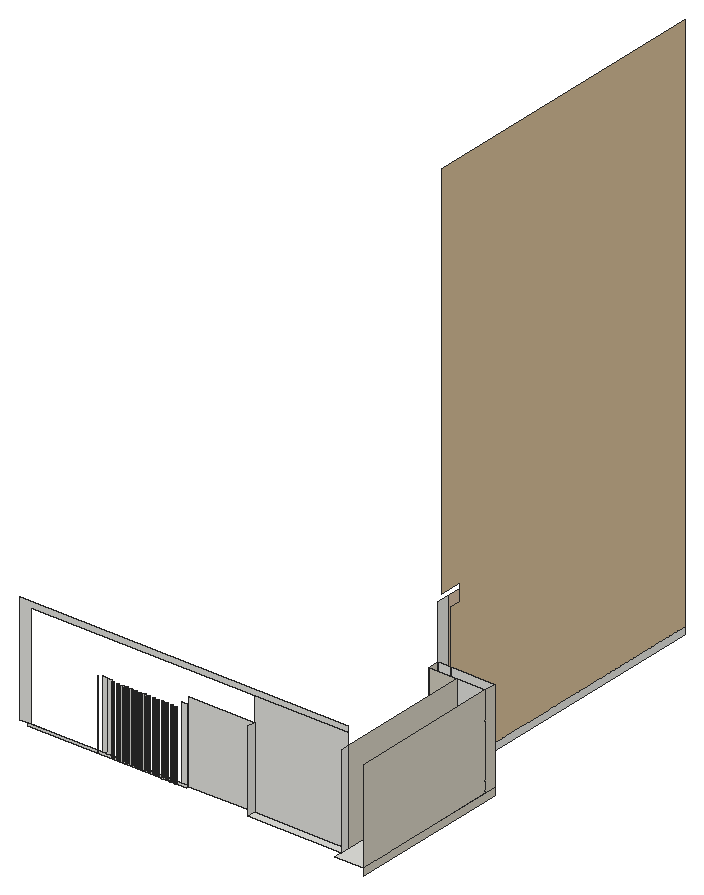
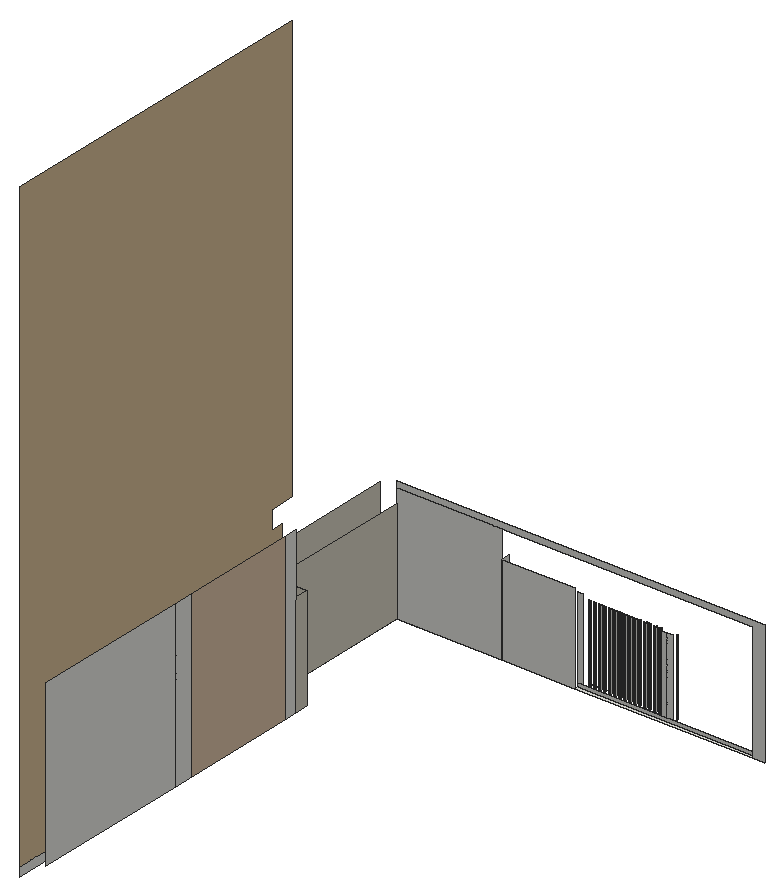
# SketchUp Ruby script. Lengths in inches.
U = 1.inch
M = Sketchup.active_model
def pt(a) = Geom::Point3d.new(a.map { |v| v * U })
def face(e, loops, mat)
  f = e.add_face(loops[0].map { |a| pt(a) })
  loops[1..].each { |l| e.add_face(l.map { |a| pt(a) }).erase! }
  f.material = f.back_material = mat if mat
  f
end
# faces: each face lists its corners as indices into pts; further lists are holes
def faces(e, pts, list, mat = nil) = list.each { |f| face(e, (f[0].is_a?(Array) ? f : [f]).map { |l| l.map { |i| pts[i] } }, mat) }
# xy, xz, yz: faces in a plane at the given z, y or x. An outline is a flat list of corners, or four numbers for a rectangle; further outlines are holes
def ring(l) = l.size == 4 ? [[l[0], l[1]], [l[2], l[1]], [l[2], l[3]], [l[0], l[3]]] : l.each_slice(2).to_a
def flat(e, list, mat, &to3) = list.each { |f| face(e, (f[0].is_a?(Array) ? f : [f]).map { |l| ring(l).map { |u, v| to3.(u, v) } }, mat) }
def xy(e, z, list, mat = nil) = flat(e, list, mat) { |x, y| [x, y, z] }
def xz(e, y, list, mat = nil) = flat(e, list, mat) { |x, z| [x, y, z] }
def yz(e, x, list, mat = nil) = flat(e, list, mat) { |y, z| [x, y, z] }
def lines(e, pts, list) = list.each { |a, b| e.add_line(pt(pts[a]), pt(pts[b])) }
# prism: a flat outline (further loops are holes) pulled along v
def prism(e, loops, v, mat = nil)
  f = face(e, loops, mat); d = Geom::Vector3d.new(v.map { |x| x * U })
  f.pushpull(f.normal.samedirection?(d) ? d.length : -d.length)
end
def box(e, o, s, mat = nil) = prism(e, [[o, [o[0] + s[0], o[1], o[2]], [o[0] + s[0], o[1] + s[1], o[2]], [o[0], o[1] + s[1], o[2]]]], [0, 0, s[2]], mat)
def at(x, y, z, deg = 0) = Geom::Transformation.translation(pt([x, y, z])) * Geom::Transformation.rotation(ORIGIN, Z_AXIS, deg.degrees)
def axes(o, x, y, z) = Geom::Transformation.new([*x, 0, *y, 0, *z, 0, *pt(o).to_a, 1])
def part(name) = M.definitions.add(name)
# library, detail: a bought-in or finely detailed component or shape, given as its bounding box
def library(name, o, s) = part(name).tap { |d| box(d.entities, o, s) }
def detail(e, o, s) = box(e.add_group.entities, o, s)
def put(e, d, t, mat = nil) = e.add_instance(d, t).tap { |i| i.material = mat if mat }
def group(e, t, mat = nil) = e.add_group.tap { |g| g.transformation = t; g.material = mat if mat }.entities
root = M.entities
M.materials.add("[Formica Beige]").color = [211, 187, 149]
M.materials.add("[Formica Graystone]").color = [209, 204, 189]
M.materials.add("[Formica Laminate Light]").color = [213, 189, 164]
xy(root,9,[[762.14,1.67,797.12,189.01],[646.62,11.52,762.14,21.38],[370.65,17.41,566.39,21.38],[727.17,189.01,797.12,203.79]])
xy(root,12.5,[[539.51,12.51,539.19,12.55,538.89,12.67,538.63,12.875,538.43,13.13,538.31,13.43,538.26,13.76,538.31,14.08,538.43,14.38,538.63,14.64,538.89,14.84,539.19,14.96,539.51,15.01,539.84,14.96,540.14,14.84,540.4,14.64,540.6,14.38,540.72,14.08,540.76,13.76,540.72,13.43,540.6,13.13,540.4,12.875,540.14,12.67,539.84,12.55],[544.76,12.51,544.44,12.55,544.14,12.67,543.88,12.875,543.68,13.13,543.56,13.43,543.51,13.76,543.56,14.08,543.68,14.38,543.88,14.64,544.14,14.84,544.44,14.96,544.76,15.01,545.09,14.96,545.39,14.84,545.65,14.64,545.85,14.38,545.97,14.08,546.01,13.76,545.97,13.43,545.85,13.13,545.65,12.875,545.39,12.67,545.09,12.55],[550.39,12.51,550.07,12.55,549.76,12.67,549.51,12.875,549.31,13.13,549.18,13.43,549.14,13.76,549.18,14.08,549.31,14.38,549.51,14.64,549.76,14.84,550.07,14.96,550.39,15.01,550.71,14.96,551.01,14.84,551.27,14.64,551.47,14.38,551.6,14.08,551.64,13.76,551.6,13.43,551.47,13.13,551.27,12.875,551.01,12.67,550.71,12.55],[555.89,12.51,555.57,12.55,555.26,12.67,555.01,12.875,554.81,13.13,554.68,13.43,554.64,13.76,554.68,14.08,554.81,14.38,555.01,14.64,555.26,14.84,555.57,14.96,555.89,15.01,556.21,14.96,556.51,14.84,556.77,14.64,556.97,14.38,557.1,14.08,557.14,13.76,557.1,13.43,556.97,13.13,556.77,12.875,556.51,12.67,556.21,12.55]])
xz(root,17.41,[[370.65,9,566.39,12.5],[462.5,12.5,468.46,96.37],[468.46,12.5,474.42,96.37],[560.77,12.5,566.39,102.25]])
xz(root,21.38,[[357.9375,9,357.9375,145.125,762.14,145.125,762.14,138.11,370.65,138.11,370.65,9],[566.39,9,646.62,108],[646.62,9,762.14,138.11]])
xz(root,189.01,[[762.14,9,797.12,122.6875]])
xz(root,189.01,[[727.17,9,762.14,122.6875]],"[Formica Graystone]")
xz(root,203.79,[[742.93,0,797.12,9],[727.17,9,742.93,122.6875],[742.93,9,797.12,122.6875]])
yz(root,646.62,[[11.52,9,21.38,108]])
yz(root,727.17,[[203.79,9,219.56,189],[348.07,9,370.07,189],[370.07,9,548.03,189]])
yz(root,727.17,[[189.01,9,203.79,122.6875]],"[Formica Graystone]")
yz(root,727.17,[[219.56,9,348.07,189]],"[Formica Laminate Light]")
yz(root,742.93,[[203.79,0,563.79,9]])
yz(root,742.93,[[203.79,9,563.79,9,563.79,679.64,190.11,679.64,190.11,209.5,218.11,209.5,218.11,189,203.79,189]],"[Formica Beige]")
yz(root,762.14,[[11.52,9,21.38,122.6875]])
yz(root,762.14,[[21.38,9,189.01,122.6875]],"[Formica Graystone]")
yz(root,797.12,[[1.67,0,203.79,9],[1.67,9,189.01,122.6875],[189.01,9,203.79,122.6875]],"[Formica Graystone]")
p = [[459.89,13.76,12.5],[459.85,14.08,12.5],[459.85,14.08,96.37],[459.89,13.76,96.37],[477.24,14.08,12.5],[477.2,13.76,12.5],
  [477.2,13.76,96.37],[477.24,14.08,96.37],[479.7,13.76,12.5],[479.66,14.08,12.5],[479.66,14.08,96.37],[479.7,13.76,96.37],
  [482.81,14.08,12.5],[482.76,13.76,12.5],[482.76,13.76,96.37],[482.81,14.08,96.37],[485.26,13.76,12.5],[485.22,14.08,12.5],
  [485.22,14.08,96.37],[485.26,13.76,96.37],[488.62,14.08,12.5],[488.58,13.76,12.5],[488.58,13.76,96.37],[488.62,14.08,96.37],
  [491.08,13.76,12.5],[491.03,14.08,12.5],[491.03,14.08,96.37],[491.08,13.76,96.37],[493.93,14.08,12.5],[493.89,13.76,12.5],
  [493.89,13.76,96.37],[493.93,14.08,96.37],[496.39,13.76,12.5],[496.35,14.08,12.5],[496.35,14.08,96.37],[496.39,13.76,96.37],
  [499.74,14.08,12.5],[499.7,13.76,12.5],[499.7,13.76,96.37],[499.74,14.08,96.37],[502.2,13.76,12.5],[502.16,14.08,12.5],
  [502.16,14.08,96.37],[502.2,13.76,96.37],[504.87,14.08,12.5],[504.83,13.76,12.5],[504.83,13.76,96.37],[504.87,14.08,96.37],
  [507.33,13.76,12.5],[507.28,14.08,12.5],[507.28,14.08,96.37],[507.33,13.76,96.37],[510.49,14.08,12.5],[510.45,13.76,12.5],
  [510.45,13.76,96.37],[510.49,14.08,96.37],[512.95,13.76,12.5],[512.91,14.08,12.5],[512.91,14.08,96.37],[512.95,13.76,96.37],
  [515.81,14.08,12.5],[515.76,13.76,12.5],[515.76,13.76,96.37],[515.81,14.08,96.37],[518.26,13.76,12.5],[518.22,14.08,12.5],
  [518.22,14.08,96.37],[518.26,13.76,96.37],[521.12,14.08,12.5],[521.08,13.76,12.5],[521.08,13.76,96.37],[521.12,14.08,96.37],
  [523.58,13.76,12.5],[523.53,14.08,12.5],[523.53,14.08,96.37],[523.58,13.76,96.37],[526.99,14.08,12.5],[526.95,13.76,12.5],
  [526.95,13.76,96.37],[526.99,14.08,96.37],[529.45,13.76,12.5],[529.41,14.08,12.5],[529.41,14.08,96.37],[529.45,13.76,96.37],
  [532.49,14.08,12.5],[532.45,13.76,12.5],[532.45,13.76,96.37],[532.49,14.08,96.37],[534.95,13.76,12.5],[534.91,14.08,12.5],
  [534.91,14.08,96.37],[534.95,13.76,96.37],[538.31,14.08,12.5],[538.26,13.76,12.5],[538.26,13.76,96.37],[538.31,14.08,96.37],
  [540.76,13.76,12.5],[540.72,14.08,12.5],[540.72,14.08,96.37],[540.76,13.76,96.37],[543.56,14.08,12.5],[543.51,13.76,12.5],
  [543.51,13.76,96.37],[543.56,14.08,96.37],[546.01,13.76,12.5],[545.97,14.08,12.5],[545.97,14.08,96.37],[546.01,13.76,96.37],
  [549.18,14.08,12.5],[549.14,13.76,12.5],[549.14,13.76,96.37],[549.18,14.08,96.37],[551.64,13.76,12.5],[551.6,14.08,12.5],
  [551.6,14.08,96.37],[551.64,13.76,96.37],[554.68,14.08,12.5],[554.64,13.76,12.5],[554.64,13.76,96.37],[554.68,14.08,96.37],
  [557.14,13.76,12.5],[557.1,14.08,12.5],[557.1,14.08,96.37],[557.14,13.76,96.37],[459.72,14.38,12.5],[459.72,14.38,96.37],
  [477.37,14.38,12.5],[477.37,14.38,96.37],[479.53,14.38,12.5],[479.53,14.38,96.37],[482.93,14.38,12.5],[482.93,14.38,96.37],
  [485.1,14.38,12.5],[485.1,14.38,96.37],[488.74,14.38,12.5],[488.74,14.38,96.37],[490.91,14.38,12.5],[490.91,14.38,96.37],
  [494.06,14.38,12.5],[494.06,14.38,96.37],[496.22,14.38,12.5],[496.22,14.38,96.37],[499.87,14.38,12.5],[499.87,14.38,96.37],
  [502.03,14.38,12.5],[502.03,14.38,96.37],[504.99,14.38,12.5],[504.99,14.38,96.37],[507.16,14.38,12.5],[507.16,14.38,96.37],
  [510.62,14.38,12.5],[510.62,14.38,96.37],[512.78,14.38,12.5],[512.78,14.38,96.37],[515.93,14.38,12.5],[515.93,14.38,96.37],
  [518.1,14.38,12.5],[518.1,14.38,96.37],[521.24,14.38,12.5],[521.24,14.38,96.37],[523.41,14.38,12.5],[523.41,14.38,96.37],
  [527.12,14.38,12.5],[527.12,14.38,96.37],[529.28,14.38,12.5],[529.28,14.38,96.37],[532.62,14.38,12.5],[532.62,14.38,96.37],
  [534.78,14.38,12.5],[534.78,14.38,96.37],[538.43,14.38,12.5],[538.43,14.38,96.37],[540.6,14.38,12.5],[540.6,14.38,96.37],
  [543.68,14.38,12.5],[543.68,14.38,96.37],[545.85,14.38,12.5],[545.85,14.38,96.37],[549.31,14.38,12.5],[549.31,14.38,96.37],
  [551.47,14.38,12.5],[551.47,14.38,96.37],[554.81,14.38,12.5],[554.81,14.38,96.37],[556.97,14.38,12.5],[556.97,14.38,96.37],
  [477.57,14.64,12.5],[477.57,14.64,96.37],[479.34,14.64,12.5],[479.34,14.64,96.37],[483.13,14.64,12.5],[483.13,14.64,96.37],
  [484.9,14.64,12.5],[484.9,14.64,96.37],[488.94,14.64,12.5],[488.94,14.64,96.37],[490.71,14.64,12.5],[490.71,14.64,96.37],
  [494.26,14.64,12.5],[494.26,14.64,96.37],[496.02,14.64,12.5],[496.02,14.64,96.37],[500.07,14.64,12.5],[500.07,14.64,96.37],
  [501.84,14.64,12.5],[501.84,14.64,96.37],[505.19,14.64,12.5],[505.19,14.64,96.37],[506.96,14.64,12.5],[506.96,14.64,96.37],
  [510.82,14.64,12.5],[510.82,14.64,96.37],[512.59,14.64,12.5],[512.59,14.64,96.37],[516.13,14.64,12.5],[516.13,14.64,96.37],
  [517.9,14.64,12.5],[517.9,14.64,96.37],[521.44,14.64,12.5],[521.44,14.64,96.37],[523.21,14.64,12.5],[523.21,14.64,96.37],
  [527.32,14.64,12.5],[527.32,14.64,96.37],[529.09,14.64,12.5],[529.09,14.64,96.37],[532.82,14.64,12.5],[532.82,14.64,96.37],
  [534.59,14.64,12.5],[534.59,14.64,96.37],[538.63,14.64,12.5],[538.63,14.64,96.37],[540.4,14.64,12.5],[540.4,14.64,96.37],
  [543.88,14.64,12.5],[543.88,14.64,96.37],[545.65,14.64,12.5],[545.65,14.64,96.37],[549.51,14.64,12.5],[549.51,14.64,96.37],
  [551.27,14.64,12.5],[551.27,14.64,96.37],[555.01,14.64,12.5],[555.01,14.64,96.37],[556.77,14.64,12.5],[556.77,14.64,96.37],
  [477.83,14.84,12.5],[477.83,14.84,96.37],[479.08,14.84,12.5],[479.08,14.84,96.37],[483.39,14.84,12.5],[483.39,14.84,96.37],
  [484.64,14.84,12.5],[484.64,14.84,96.37],[489.2,14.84,12.5],[489.2,14.84,96.37],[490.45,14.84,12.5],[490.45,14.84,96.37],
  [494.51,14.84,12.5],[494.51,14.84,96.37],[495.76,14.84,12.5],[495.76,14.84,96.37],[500.33,14.84,12.5],[500.33,14.84,96.37],
  [501.58,14.84,12.5],[501.58,14.84,96.37],[505.45,14.84,12.5],[505.45,14.84,96.37],[506.7,14.84,12.5],[506.7,14.84,96.37],
  [511.08,14.84,12.5],[511.08,14.84,96.37],[512.33,14.84,12.5],[512.33,14.84,96.37],[516.39,14.84,12.5],[516.39,14.84,96.37],
  [517.64,14.84,12.5],[517.64,14.84,96.37],[521.7,14.84,12.5],[521.7,14.84,96.37],[522.95,14.84,12.5],[522.95,14.84,96.37],
  [527.58,14.84,12.5],[527.58,14.84,96.37],[528.83,14.84,12.5],[528.83,14.84,96.37],[533.08,14.84,12.5],[533.08,14.84,96.37],
  [534.33,14.84,12.5],[534.33,14.84,96.37],[538.89,14.84,12.5],[538.89,14.84,96.37],[540.14,14.84,12.5],[540.14,14.84,96.37],
  [544.14,14.84,12.5],[544.14,14.84,96.37],[545.39,14.84,12.5],[545.39,14.84,96.37],[549.76,14.84,12.5],[549.76,14.84,96.37],
  [551.01,14.84,12.5],[551.01,14.84,96.37],[555.26,14.84,12.5],[555.26,14.84,96.37],[556.51,14.84,12.5],[556.51,14.84,96.37],
  [478.13,14.96,12.5],[478.13,14.96,96.37],[478.78,14.96,12.5],[478.78,14.96,96.37],[483.69,14.96,12.5],[483.69,14.96,96.37],
  [484.34,14.96,12.5],[484.34,14.96,96.37],[489.5,14.96,12.5],[489.5,14.96,96.37],[490.15,14.96,12.5],[490.15,14.96,96.37],
  [494.82,14.96,12.5],[494.82,14.96,96.37],[495.46,14.96,12.5],[495.46,14.96,96.37],[500.63,14.96,12.5],[500.63,14.96,96.37],
  [501.28,14.96,12.5],[501.28,14.96,96.37],[505.75,14.96,12.5],[505.75,14.96,96.37],[506.4,14.96,12.5],[506.4,14.96,96.37],
  [511.38,14.96,12.5],[511.38,14.96,96.37],[512.03,14.96,12.5],[512.03,14.96,96.37],[516.69,14.96,12.5],[516.69,14.96,96.37],
  [517.34,14.96,12.5],[517.34,14.96,96.37],[522,14.96,12.5],[522,14.96,96.37],[522.65,14.96,12.5],[522.65,14.96,96.37],
  [527.88,14.96,12.5],[527.88,14.96,96.37],[528.53,14.96,12.5],[528.53,14.96,96.37],[533.38,14.96,12.5],[533.38,14.96,96.37],
  [534.03,14.96,12.5],[534.03,14.96,96.37],[539.19,14.96,12.5],[539.19,14.96,96.37],[539.84,14.96,12.5],[539.84,14.96,96.37],
  [544.44,14.96,12.5],[544.44,14.96,96.37],[545.09,14.96,12.5],[545.09,14.96,96.37],[550.07,14.96,12.5],[550.07,14.96,96.37],
  [550.71,14.96,12.5],[550.71,14.96,96.37],[555.57,14.96,12.5],[555.57,14.96,96.37],[556.21,14.96,12.5],[556.21,14.96,96.37],
  [478.45,15.01,12.5],[478.45,15.01,96.37],[484.01,15.01,12.5],[484.01,15.01,96.37],[489.83,15.01,12.5],[489.83,15.01,96.37],
  [495.14,15.01,12.5],[495.14,15.01,96.37],[500.95,15.01,12.5],[500.95,15.01,96.37],[506.08,15.01,12.5],[506.08,15.01,96.37],
  [511.7,15.01,12.5],[511.7,15.01,96.37],[517.01,15.01,12.5],[517.01,15.01,96.37],[522.33,15.01,12.5],[522.33,15.01,96.37],
  [528.2,15.01,12.5],[528.2,15.01,96.37],[533.7,15.01,12.5],[533.7,15.01,96.37],[539.51,15.01,12.5],[539.51,15.01,96.37],
  [544.76,15.01,12.5],[544.76,15.01,96.37],[550.39,15.01,12.5],[550.39,15.01,96.37],[555.89,15.01,12.5],[555.89,15.01,96.37]]
faces(root,p,[[0,1,2,3],[4,5,6,7],[8,9,10,11],[12,13,14,15],[16,17,18,19],[20,21,22,23],[24,25,26,27],[28,29,30,31],
  [32,33,34,35],[36,37,38,39],[40,41,42,43],[44,45,46,47],[48,49,50,51],[52,53,54,55],[56,57,58,59],[60,61,62,63],
  [64,65,66,67],[68,69,70,71],[72,73,74,75],[76,77,78,79],[80,81,82,83],[84,85,86,87],[88,89,90,91],[92,93,94,95],
  [96,97,98,99],[100,101,102,103],[104,105,106,107],[108,109,110,111],[112,113,114,115],[116,117,118,119],[120,121,122,123],[1,124,125,2],
  [126,4,7,127],[9,128,129,10],[130,12,15,131],[17,132,133,18],[134,20,23,135],[25,136,137,26],[138,28,31,139],[33,140,141,34],
  [142,36,39,143],[41,144,145,42],[146,44,47,147],[49,148,149,50],[150,52,55,151],[57,152,153,58],[154,60,63,155],[65,156,157,66],
  [158,68,71,159],[73,160,161,74],[162,76,79,163],[81,164,165,82],[166,84,87,167],[89,168,169,90],[170,92,95,171],[97,172,173,98],
  [174,100,103,175],[105,176,177,106],[178,108,111,179],[113,180,181,114],[182,116,119,183],[121,184,185,122],[186,126,127,187],[128,188,189,129],
  [190,130,131,191],[132,192,193,133],[194,134,135,195],[136,196,197,137],[198,138,139,199],[140,200,201,141],[202,142,143,203],[144,204,205,145],
  [206,146,147,207],[148,208,209,149],[210,150,151,211],[152,212,213,153],[214,154,155,215],[156,216,217,157],[218,158,159,219],[160,220,221,161],
  [222,162,163,223],[164,224,225,165],[226,166,167,227],[168,228,229,169],[230,170,171,231],[172,232,233,173],[234,174,175,235],[176,236,237,177],
  [238,178,179,239],[180,240,241,181],[242,182,183,243],[184,244,245,185],[246,186,187,247],[188,248,249,189],[250,190,191,251],[192,252,253,193],
  [254,194,195,255],[196,256,257,197],[258,198,199,259],[200,260,261,201],[262,202,203,263],[204,264,265,205],[266,206,207,267],[208,268,269,209],
  [270,210,211,271],[212,272,273,213],[274,214,215,275],[216,276,277,217],[278,218,219,279],[220,280,281,221],[282,222,223,283],[224,284,285,225],
  [286,226,227,287],[228,288,289,229],[290,230,231,291],[232,292,293,233],[294,234,235,295],[236,296,297,237],[298,238,239,299],[240,300,301,241],
  [302,242,243,303],[244,304,305,245],[306,246,247,307],[248,308,309,249],[310,250,251,311],[252,312,313,253],[314,254,255,315],[256,316,317,257],
  [318,258,259,319],[260,320,321,261],[322,262,263,323],[264,324,325,265],[326,266,267,327],[268,328,329,269],[330,270,271,331],[272,332,333,273],
  [334,274,275,335],[276,336,337,277],[338,278,279,339],[280,340,341,281],[342,282,283,343],[284,344,345,285],[346,286,287,347],[288,348,349,289],
  [350,290,291,351],[292,352,353,293],[354,294,295,355],[296,356,357,297],[358,298,299,359],[300,360,361,301],[362,302,303,363],[304,364,365,305],
  [366,306,307,367],[308,366,367,309],[368,310,311,369],[312,368,369,313],[370,314,315,371],[316,370,371,317],[372,318,319,373],[320,372,373,321],
  [374,322,323,375],[324,374,375,325],[376,326,327,377],[328,376,377,329],[378,330,331,379],[332,378,379,333],[380,334,335,381],[336,380,381,337],
  [382,338,339,383],[340,382,383,341],[384,342,343,385],[344,384,385,345],[386,346,347,387],[348,386,387,349],[388,350,351,389],[352,388,389,353],
  [390,354,355,391],[356,390,391,357],[392,358,359,393],[360,392,393,361],[394,362,363,395],[364,394,395,365]])
